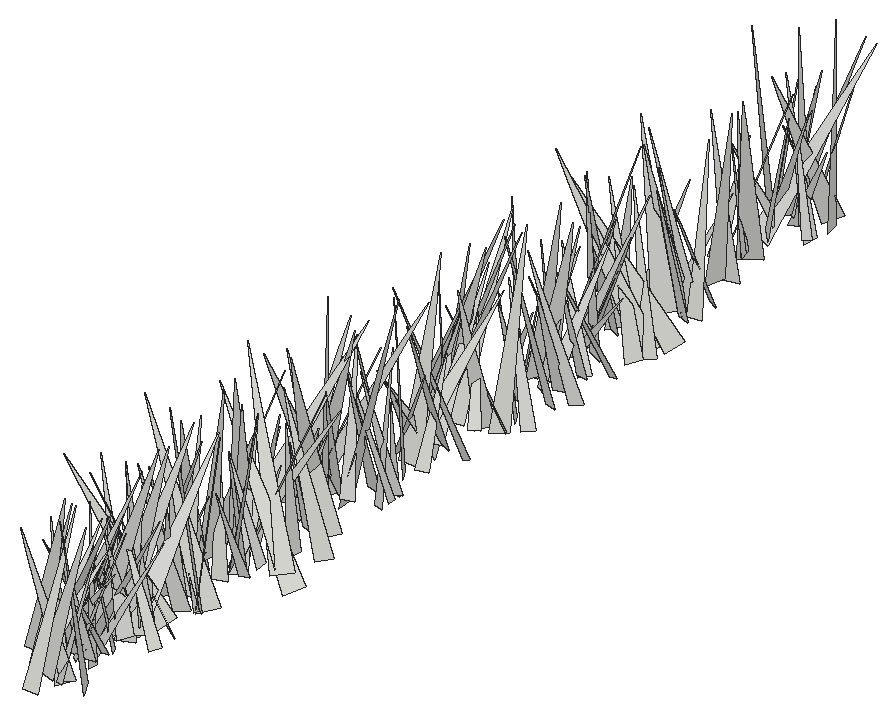
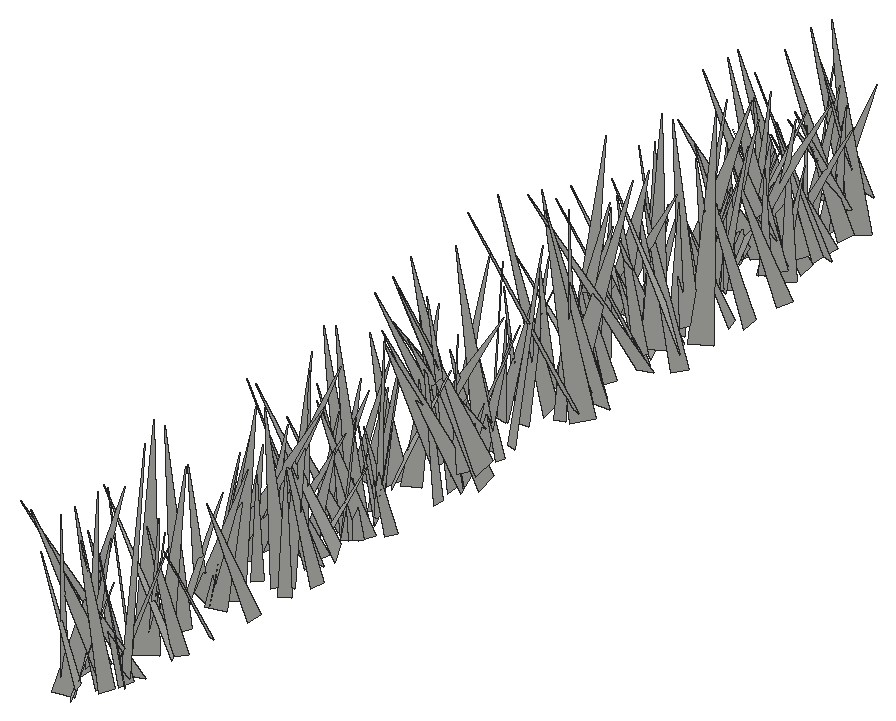
# SketchUp Ruby script. Lengths in inches.
U = 1.inch
M = Sketchup.active_model
def pt(a) = Geom::Point3d.new(a.map { |v| v * U })
def face(e, loops, mat)
  f = e.add_face(loops[0].map { |a| pt(a) })
  loops[1..].each { |l| e.add_face(l.map { |a| pt(a) }).erase! }
  f.material = f.back_material = mat if mat
  f
end
# faces: each face lists its corners as indices into pts; further lists are holes
def faces(e, pts, list, mat = nil) = list.each { |f| face(e, (f[0].is_a?(Array) ? f : [f]).map { |l| l.map { |i| pts[i] } }, mat) }
# xy, xz, yz: faces in a plane at the given z, y or x. An outline is a flat list of corners, or four numbers for a rectangle; further outlines are holes
def ring(l) = l.size == 4 ? [[l[0], l[1]], [l[2], l[1]], [l[2], l[3]], [l[0], l[3]]] : l.each_slice(2).to_a
def flat(e, list, mat, &to3) = list.each { |f| face(e, (f[0].is_a?(Array) ? f : [f]).map { |l| ring(l).map { |u, v| to3.(u, v) } }, mat) }
def xy(e, z, list, mat = nil) = flat(e, list, mat) { |x, y| [x, y, z] }
def xz(e, y, list, mat = nil) = flat(e, list, mat) { |x, z| [x, y, z] }
def yz(e, x, list, mat = nil) = flat(e, list, mat) { |y, z| [x, y, z] }
def lines(e, pts, list) = list.each { |a, b| e.add_line(pt(pts[a]), pt(pts[b])) }
# prism: a flat outline (further loops are holes) pulled along v
def prism(e, loops, v, mat = nil)
  f = face(e, loops, mat); d = Geom::Vector3d.new(v.map { |x| x * U })
  f.pushpull(f.normal.samedirection?(d) ? d.length : -d.length)
end
def box(e, o, s, mat = nil) = prism(e, [[o, [o[0] + s[0], o[1], o[2]], [o[0] + s[0], o[1] + s[1], o[2]], [o[0], o[1] + s[1], o[2]]]], [0, 0, s[2]], mat)
def at(x, y, z, deg = 0) = Geom::Transformation.translation(pt([x, y, z])) * Geom::Transformation.rotation(ORIGIN, Z_AXIS, deg.degrees)
def axes(o, x, y, z) = Geom::Transformation.new([*x, 0, *y, 0, *z, 0, *pt(o).to_a, 1])
def part(name) = M.definitions.add(name)
# library, detail: a bought-in or finely detailed component or shape, given as its bounding box
def library(name, o, s) = part(name).tap { |d| box(d.entities, o, s) }
def detail(e, o, s) = box(e.add_group.entities, o, s)
def put(e, d, t, mat = nil) = e.add_instance(d, t).tap { |i| i.material = mat if mat }
def group(e, t, mat = nil) = e.add_group.tap { |g| g.transformation = t; g.material = mat if mat }.entities
root = M.entities
c1 = part("fur_instance\#9")
p = [[0.8125,0,1.79],[0.67,-0.02,1.48],[0,-0.11,0],[0,0.11,0]]
faces(c1.entities,p,[[0,1,2,3]])
put(root,c1,axes([155.28,108.74,-27.1],[0.56131,-6.10589,2.64479],[-6.41112,0.21442,1.85565],[1.78167,2.69518,5.8441]))
put(root,c1,axes([156,106.33,-27.1],[0.77683,6.56918,0.32302],[6.56801,-0.79193,0.30978],[-0.34589,-0.28401,6.60769]))
put(root,c1,axes([157.04,109.05,-27.1],[-1.11932,5.12608,2.18052],[5.30702,0.30525,2.00664],[-1.6932,-2.43194,4.84799]))
put(root,c1,axes([157.4,110.48,-28.22],[-5.52938,-3.456,2.07939],[-3.45701,5.87854,0.57763],[2.07771,0.58365,6.49494]))
put(root,c1,axes([152.8,110.96,-27.1],[2.44609,-6.94499,1.47158],[-6.99231,-2.08787,1.76924],[1.22722,1.94671,7.14745]))
put(root,c1,axes([154.06,109.06,-27.1],[2.83544,5.2975,1.05869],[5.3487,-2.92083,0.29014],[-0.75876,-0.79328,6.00159]))
put(root,c1,axes([156.75,108.45,-27.1],[2.63197,4.07891,0.20518],[3.86496,-2.5665,1.44292],[-1.31973,0.61842,4.63495]))
put(root,c1,axes([155.76,110.05,-28.22],[-5.59826,1.4556,0.99849],[1.35798,5.67289,-0.65612],[1.12768,0.39476,5.74707]))
put(root,c1,axes([155.02,112.17,-27.1],[-0.84306,-4.44176,0.86686],[-4.52258,0.85891,0.00263],[0.16427,0.85115,4.52106]))
put(root,c1,axes([154.27,109.05,-27.1],[-0.54715,4.89077,0.10405],[4.53126,0.54616,-1.84371],[1.84341,0.10915,4.56287]))
put(root,c1,axes([156.3125,112.18,-27.1],[0.08099,-5.17118,1.20761],[-5.27072,-0.22549,-0.61212],[-0.64729,1.18913,5.13546]))
put(root,c1,axes([153.21,111.98,-27.1],[6.75875,-1.16964,0.00047],[-1.16859,-6.75255,0.29358],[0.0496,0.28936,6.85293]))
put(root,c1,axes([153.85,110.38,-27.1],[-1.09311,5.26549,0.63584],[5.05113,1.23151,-1.51458],[1.61731,-0.28736,5.16007]))
put(root,c1,axes([156.67,113.47,-27.1],[-1.81586,-4.37557,0.34615],[-4.20637,1.62778,-1.48984],[-1.25376,0.87607,4.49704]))
put(root,c1,axes([155.61,111.54,-27.1],[3.29969,3.36632,0.10349],[3.25213,-3.22241,1.12716],[-0.87548,0.71745,4.57707]))
put(root,c1,axes([155.58,112.52,-27.1],[3.89268,2.82638,0.90518],[2.67493,-3.98806,0.94914],[-1.28551,0.26015,4.71599]))
put(root,c1,axes([152.82,113.93,-27.1],[2.65844,-2.5721,0.0216],[-2.2994,-2.3625,1.67773],[1.15278,1.21916,3.2967]))
put(root,c1,axes([155.84,113.16,-28.22],[-5.50715,-0.70612,1.61288],[-1.08889,5.52799,-1.29784],[1.38358,1.53996,5.39842]))
put(root,c1,axes([155.6,115.7,-28.22],[-3.07283,-1.79032,0.75021],[-1.87261,3.10397,-0.26279],[0.51124,0.60869,3.54662]))
put(root,c1,axes([152.41,114.9,-27.1],[3.65176,6.04586,1.11201],[6.02251,-3.25936,-2.05677],[1.23222,-1.98709,6.75703]))
put(root,c1,axes([152.82,115.48,-27.1],[5.19271,0.37939,0.34653],[0.38191,-5.20401,-0.02543],[-0.34375,-0.05067,5.20649]))
put(root,c1,axes([154.72,114.96,-28.22],[3.55975,3.91646,0.08522],[3.79537,-3.41954,-1.38552],[0.97011,-0.99289,5.10792]))
put(root,c1,axes([155.55,117.68,-28.22],[3.33283,-3.55166,1.19436],[-3.37517,-3.53973,-1.10774],[-1.62758,0.06765,4.74288]))
put(root,c1,axes([158.9375,115.97,-27.1],[-4.27711,1.68369,0.0136],[1.68167,4.26988,0.26227],[-0.08344,-0.24902,4.58909]))
put(root,c1,axes([154.35,117.61,-28.22],[-3.58815,0.95471,1.93369],[1.59157,3.70529,1.12394],[1.45517,-1.69849,3.5388]))
put(root,c1,axes([153.92,116.01,-27.1],[6.10397,-4.61293,1.81963],[-4.95361,-5.80478,1.9013],[-0.22786,2.62185,7.41098]))
put(root,c1,axes([153.81,115.41,-28.22],[5.39304,-0.33096,0.39775],[-0.43435,-5.15892,1.59671],[-0.28121,1.6213,5.16187]))
put(root,c1,axes([153.73,117.42,-28.22],[3.93082,-2.70083,1.38603],[-2.7651,-4.12134,-0.18897],[-1.2529,0.6221,4.76552]))
put(root,c1,axes([156.42,115.96,-27.1],[-6.22467,1.67352,0.58559],[1.62437,6.23957,-0.56507],[0.71064,0.39649,6.42089]))
put(root,c1,axes([155.38,117.21,-28.22],[3.4619,-5.09824,2.22403],[-5.52391,-3.4582,0.67108],[-0.65172,2.22978,6.12588]))
put(root,c1,axes([157.35,119.18,-27.1],[-6.27712,3.42033,1.55819],[3.73626,5.34865,3.31076],[-0.40863,-3.63622,6.33559]))
put(root,c1,axes([156.74,117.86,-27.1],[5.59524,-0.57904,3.08549],[-0.36766,-6.38318,-0.53118],[-3.11775,-0.28642,5.59999]))
put(root,c1,axes([157.17,119.92,-28.22],[-4.1792,-5.61615,0.15739],[-5.61189,4.16336,-0.45249],[-0.26934,0.3962,6.98585]))
put(root,c1,axes([156.85,119.97,-27.1],[-4.22388,-0.55824,1.0602],[-0.01996,3.91714,1.98304],[1.19803,-1.90295,3.77099]))
put(root,c1,axes([154,118.47,-27.1],[4.37755,-6.1842,1.75356],[-6.40379,-4.01166,1.83857],[0.55746,2.47882,7.3503]))
put(root,c1,axes([156.9,116.99,-27.1],[-0.83276,5.81039,0.96307],[5.68734,0.54058,1.65638],[-1.53047,-1.15272,5.63121]))
put(root,c1,axes([154.28,119.24,-27.1],[-2.72992,2.63061,1.69887],[2.87463,2.99911,-0.02472],[1.24209,-1.1593,3.79104]))
put(root,c1,axes([154.4,117.78,-27.1],[-0.17327,7.80384,1.95788],[7.72096,0.71202,-2.15474],[2.26272,-1.83203,7.50246]))
put(root,c1,axes([152,120.01,-28.22],[4.26333,-3.02404,0.31767],[-2.97687,-4.03955,1.49732],[0.61963,1.39963,5.00788]))
put(root,c1,axes([156.96,121.24,-27.1],[0.96308,-5.75121,1.64983],[-5.7805,-1.32563,-1.24675],[-1.54408,1.37555,5.69645]))
put(root,c1,axes([155.87,117.6,-27.1],[-2.00066,7.03095,0.19663],[6.73059,1.97306,-2.06922],[2.04255,0.38513,7.01108]))
put(root,c1,axes([154.93,122.35,-27.1],[3.91329,-2.80057,0.16354],[-2.76188,-3.89534,-0.61821],[-0.49189,-0.40864,4.7723]))
put(root,c1,axes([155.8,122.39,-27.1],[1.04102,-4.92803,1.21287],[-5.07408,-1.03535,0.14838],[-0.10125,1.21771,5.0346]))
put(root,c1,axes([155.33,122.57,-27.1],[-1.95958,-4.83915,1.26512],[-4.97855,2.01787,0.00704],[0.48156,1.1699,5.22085]))
put(root,c1,axes([157.79,122.03,-27.1],[-4.59653,-5.39297,2.39685],[-5.86856,4.49796,-1.13384],[0.62378,2.57709,6.99476]))
put(root,c1,axes([158.34,122.38,-27.1],[-5.06971,5.94983,1.91077],[6.22333,4.58369,2.23904],[-0.56711,-2.88838,7.48926]))
put(root,c1,axes([157.86,121.75,-27.1],[-3.7674,-0.4134,0.34529],[-0.49063,3.64055,-0.99453],[0.22227,1.02903,3.6572]))
put(root,c1,axes([156.02,125.67,-28.22],[-5.03232,-2.4099,0.87584],[-1.92345,4.82363,2.22078],[1.6956,-1.68045,5.11859]))
put(root,c1,axes([152.14,123.56,-28.22],[6.68807,0.43229,0.66728],[0.41432,-6.71942,0.20043],[-0.67859,0.15798,6.69903]))
put(root,c1,axes([155.62,125.4,-27.1],[-2.21382,-3.77344,0.32599],[-3.76288,2.23425,0.30817],[0.43109,0.1241,4.36404]))
put(root,c1,axes([155.875,123.06,-27.1],[0.35449,6.1752,1.09899],[6.2119,-0.49795,0.79425],[-0.86782,-1.04187,6.13416]))
put(root,c1,axes([154.59,125.72,-28.22],[3.69815,0.46024,1.83595],[1.02421,-3.87534,-1.09159],[-1.5917,-1.42435,3.56322]))
put(root,c1,axes([153.07,124.3,-28.22],[3.9948,0.59542,0.26899],[0.55235,-3.96784,0.58004],[-0.34899,0.53573,3.99706]))
put(root,c1,axes([156.08,123.89,-28.22],[4.62309,3.63215,1.82021],[3.50208,-4.96051,1.00367],[-2.05939,-0.28182,5.79293]))
put(root,c1,axes([153.02,127.67,-28.22],[4.3126,-6.65441,0.44802],[-6.65528,-4.32849,-0.22777],[-0.435,0.25174,7.9264]))
put(root,c1,axes([157.32,127.48,-27.1],[0.58704,-3.79537,0.45103],[-3.78334,-0.64184,-0.47675],[-0.5428,0.36891,3.81079]))
put(root,c1,axes([153.91,127.75,-27.1],[6.97924,-1.80721,1.76653],[-1.77915,-7.19853,-0.33521],[-1.79479,0.10824,7.20163]))
put(root,c1,axes([155.84,128.07,-27.1],[5.68987,2.39384,1.65752],[2.61602,-5.80047,-0.60296],[-1.2784,-1.21517,6.14342]))
put(root,c1,axes([155.09,127.64,-28.22],[-1.15441,5.11883,1.74969],[5.40957,1.09949,0.35248],[0.0216,-1.78472,5.23554]))
put(root,c1,axes([156.03,128.94,-27.1],[-1.67476,-3.89018,1.26522],[-4.03938,1.78862,0.15259],[0.64624,1.09838,4.23261]))
put(root,c1,axes([157.33,129.25,-27.1],[-4.29082,0.07848,0.62907],[0.12494,4.3243,0.31276],[0.62151,-0.32753,4.28013]))
put(root,c1,axes([153.75,131.74,-27.1],[4.25947,-6.86655,0.67935],[-6.89421,-4.26807,0.08653],[-0.2843,0.62304,8.07992]))
put(root,c1,axes([154.02,131.65,-27.1],[3.44417,-6.15496,0.43731],[-6.17002,-3.42915,0.33004],[0.07525,0.54268,7.04535]))
put(root,c1,axes([159.93,129.55,-28.22],[-5.28258,5.45364,0.12335],[5.18528,4.96674,2.47132],[-1.69419,-1.80343,7.17917]))
put(root,c1,axes([155.55,129.04,-28.22],[3.74309,-3.05687,3.19875],[-4.02453,-4.09315,0.7978],[-1.83838,2.73658,4.76642]))
put(root,c1,axes([151.78,131.4375,-28.22],[2.36521,-5.47601,0.71506],[-5.30162,-2.03369,1.96193],[1.54624,1.40343,5.6331]))
put(root,c1,axes([159.06,129.3125,-27.1],[-3.56857,7.17935,0.49748],[7.02506,3.35468,1.97986],[-1.56176,-1.31463,7.76903]))
put(root,c1,axes([155.07,129.56,-28.22],[-2.46279,4.53865,0.90199],[4.34757,2.61941,-1.3098],[1.58479,-0.13272,4.99491]))
put(root,c1,axes([152.375,130.54,-27.1],[6.025,3.41302,0.55167],[3.40656,-6.04972,0.22351],[-0.59027,-0.07668,6.92094]))
put(root,c1,axes([154.72,130.52,-28.22],[6.48449,2.8801,0.19854],[2.8437,-6.45643,0.78158],[-0.49773,0.63448,7.05214]))
put(root,c1,axes([153.87,133,-27.1],[5.53978,-0.90724,0.62547],[-0.85463,-5.56113,-0.49688],[-0.69563,-0.39269,5.59154]))
put(root,c1,axes([156.8125,133.34,-28.22],[-4.81176,0.83188,2.6308],[1.27412,5.3609,0.63523],[2.44739,-1.15538,4.84165]))
put(root,c1,axes([154.01,132.54,-28.22],[2.6099,-2.39325,0.8726],[-2.54736,-2.4537,0.88934],[-0.00348,1.24593,3.42758]))
put(root,c1,axes([153.79,133.01,-27.1],[3.84668,4.92623,0.09388],[4.62666,-3.57049,-2.21792],[1.69428,-1.43435,5.84342]))
put(root,c1,axes([158.85,134.08,-28.22],[-2.40654,5.51072,1.54274],[5.60544,1.9331,1.83892],[-1.15197,-2.10585,5.72519]))
put(root,c1,axes([155.44,137.81,-27.1],[6.81384,-4.6319,0.82302],[-4.34734,-6.75311,-2.01405],[-1.7979,-1.22528,7.98915]))
put(root,c1,axes([155.24,136.69,-28.22],[-0.97443,-3.66118,0.75209],[-3.71136,1.03977,0.25308],[0.44234,0.6588,3.78017]))
put(root,c1,axes([157.17,136.85,-28.22],[3.76435,-5.16952,3.38659],[-5.24976,-4.76711,-1.44149],[-3.26082,1.70703,6.23028]))
put(root,c1,axes([154.72,139.375,-27.1],[4.80853,-5.64104,1.01196],[-5.19564,-4.8483,-2.3381],[-2.41883,-0.80002,7.03396]))
put(root,c1,axes([153.22,137.09,-27.1],[3.00481,-2.76961,0.12717],[-2.71494,-2.90128,0.96303],[0.56213,0.79222,3.97142]))
put(root,c1,axes([153.6,137.51,-28.22],[0.78956,-4.05986,1.16414],[-3.93825,-0.27989,1.69498],[1.52574,1.37851,3.77266]))
put(root,c1,axes([152.41,134.41,-27.1],[1.49345,8.09623,0.02611],[7.76227,-1.42429,-2.34489],[2.30146,-0.44999,7.89182]))
put(root,c1,axes([154.35,138.95,-28.22],[1.6475,-3.20979,0.84583],[-3.31321,-1.64761,0.20101],[-0.20196,0.8456,3.6023]))
put(root,c1,axes([155.5,138.28,-27.1],[-6.71268,-1.89599,2.76742],[-2.51748,6.93875,-1.3526],[2.21714,2.13833,6.8429]))
put(root,c1,axes([152.88,138.43,-28.22],[1.96643,7.28816,1.86053],[7.47956,-1.69089,-1.28167],[0.79683,-2.11408,7.43918]))
put(root,c1,axes([153.86,141.6875,-28.22],[-0.85203,-5.57664,0.61964],[-5.3803,0.98986,1.51043],[1.59225,0.36067,5.43539]))
put(root,c1,axes([152.62,140.74,-28.22],[6.79044,-4.4332,0.71146],[-4.48312,-6.76549,0.63187],[-0.24718,0.91888,8.0848]))
put(root,c1,axes([153.88,137.39,-28.22],[5.76242,3.50846,0.12226],[3.39302,-5.62636,1.53663],[-0.90093,1.2508,6.56914]))
put(root,c1,axes([156.21,139.82,-27.1],[-0.40963,5.6712,0.85204],[5.69515,0.30195,0.72827],[-0.67361,-0.89587,5.63914]))
put(root,c1,axes([155.49,143.62,-28.22],[-0.77388,-5.77446,0.46112],[-5.72229,0.83441,0.84559],[0.90132,0.33953,5.76439]))
put(root,c1,axes([155.2,140.97,-28.22],[8.05424,1.38868,1.7961],[1.29513,-8.24767,0.56905],[-1.86468,0.26973,8.15325]))
put(root,c1,axes([158.61,141.58,-27.1],[-4.94313,-1.68267,0.02369],[-1.64372,4.81198,-1.18726],[-0.36076,1.13137,5.08492]))
put(root,c1,axes([152.75,141.45,-27.1],[4.68977,6.59581,0.10077],[6.41242,-4.52929,-1.96857],[1.54784,-1.22048,7.85006]))
put(root,c1,axes([157.07,143.95,-28.22],[0.47741,-4.86513,1.33169],[-4.92648,-0.73691,-0.92606],[-1.08291,1.20759,4.79999]))
put(root,c1,axes([157.14,141.98,-28.22],[2.35955,4.93164,1.36493],[4.86886,-2.62618,1.07189],[-1.57426,-0.73054,5.36093]))
put(root,c1,axes([156.96,144.05,-28.22],[-0.48209,-3.49328,1.24378],[-3.69826,0.54426,0.09516],[0.26993,1.21786,3.5251]))
put(root,c1,axes([154.15,146.48,-28.22],[-3.66849,-5.82093,1.22872],[-5.44278,3.86666,2.06783],[2.40191,-0.1285,6.56241]))
put(root,c1,axes([157.07,144.8125,-27.1],[-5.34444,-2.84039,2.21318],[-3.30562,5.4408,-0.99979],[1.42788,1.96442,5.96919]))
put(root,c1,axes([156.45,149.73,-27.1],[-1.98153,-6.18192,0.39554],[-6.00617,2.01899,1.46585],[1.5161,-0.08133,6.32408]))
put(root,c1,axes([154.42,149.6,-28.22],[3.43107,-2.8474,0.0502],[-2.64084,-3.2106,-1.6126],[-1.06592,-1.21113,4.15686]))
put(root,c1,axes([155.6,150.16,-28.22],[-4.54437,-2.07997,0.71062],[-1.49312,4.11891,2.50752],[1.61302,-2.04715,4.32318]))
put(root,c1,axes([153.6,148.31,-28.22],[4.55769,0.07164,0.01251],[0.0727,-4.46545,-0.91231],[0.00209,-0.91239,4.46602]))
put(root,c1,axes([155.19,147.89,-28.22],[-0.77106,7.66776,2.67234],[8.04873,1.0768,-0.76736],[1.07416,-2.56446,7.66813]))
put(root,c1,axes([156.35,147.61,-28.22],[-1.99149,3.68652,0.84504],[3.6319,2.13053,-0.73532],[1.05538,-0.37542,4.12502]))
put(root,c1,axes([158.9375,149.14,-27.1],[-3.53185,-5.19128,1.06072],[-4.89285,2.7062,-3.04713],[-2.03336,2.50511,5.48984]))
put(root,c1,axes([155.11,148.36,-27.1],[-2.23637,5.81255,0.47787],[5.16217,2.21098,-2.73477],[2.71405,0.58421,5.59536]))
put(root,c1,axes([155.06,150.27,-27.1],[0.14678,4.73777,0.12743],[4.7339,-0.15274,0.22615],[-0.23006,-0.12022,4.73465]))
put(root,c1,axes([154.84,151.95,-27.1],[-3.59286,-3.26733,2.03566],[-3.70516,3.69058,-0.61592],[1.04455,1.85261,4.81713]))
put(root,c1,axes([153.31,152.77,-28.22],[3.4231,3.63538,1.50249],[3.93251,-3.11512,-1.42212],[0.09387,-2.06666,4.78656]))
put(root,c1,axes([153.35,153.07,-27.1],[6.11915,-4.70581,1.11272],[-4.83462,-5.98952,1.25659],[-0.09634,1.67568,7.61641]))
put(root,c1,axes([155.83,149.45,-27.1],[-4.8564,4.18897,0.42907],[3.70643,4.56321,-2.59917],[1.99849,1.71635,5.86314]))
put(root,c1,axes([156.01,154.84,-28.22],[4.71186,-4.25626,1.34995],[-4.06485,-4.9009,-1.26409],[-1.848,-0.07223,6.22249]))
put(root,c1,axes([152.31,151.41,-28.22],[8.13769,0.92636,1.08085],[0.65484,-8.00564,1.93114],[-1.26395,1.81658,7.95932]))
put(root,c1,axes([152.52,151.4375,-27.1],[8.0865,0.10169,1.15451],[-0.2162,-7.86244,2.20681],[-1.13864,2.21504,7.78021]))
put(root,c1,axes([153.6,153.15,-28.22],[7.00703,0.38351,2.14023],[0.30488,-7.32356,0.31416],[-2.15283,0.21111,7.01048]))
put(root,c1,axes([156.87,152.54,-27.1],[-2.11834,3.44874,0.2067],[3.45458,2.11778,0.0692],[0.04913,-0.21236,4.04678]))
put(root,c1,axes([154.38,151.59,-27.1],[7.47336,0.82298,1.26079],[0.38429,-7.21504,2.43175],[-1.45575,2.3203,7.11442]))
put(root,c1,axes([153.21,155.42,-28.22],[6.22131,1.299,1.34326],[1.60809,-6.10017,-1.54868],[-0.95174,-1.81575,6.1639]))
put(root,c1,axes([157.22,155.47,-28.22],[-3.79986,-3.34827,0.10157],[-3.34083,3.7767,-0.4853],[-0.24505,0.43103,5.04126]))
put(root,c1,axes([153.34,152.29,-28.22],[7.3603,1.92647,1.4977],[1.22652,-7.03518,3.02165],[-2.10951,2.63124,6.98247]))
put(root,c1,axes([155.12,152.48,-27.1],[-6.41092,4.00729,0.82453],[3.32918,6.00061,-3.27831],[2.37798,2.40258,6.81256]))
put(root,c1,axes([157.08,154.9375,-28.22],[-6.19625,3.45387,1.64148],[3.0912,6.3638,-1.72156],[2.25127,0.76815,6.88178]))
put(root,c1,axes([156.95,156.92,-28.22],[-4.18009,-2.38384,1.39005],[-2.61185,4.23208,-0.59649],[0.8906,1.22265,4.77494]))
put(root,c1,axes([155.72,159.07,-28.22],[0.47232,-5.02453,0.37853],[-5.03579,-0.45765,0.20889],[0.17316,0.39615,5.04235]))
put(root,c1,axes([158.5,156.3,-28.22],[-1.63602,4.97918,0.62205],[4.87533,1.42244,1.43652],[-1.18757,-1.0199,5.04036]))
put(root,c1,axes([157.61,159.76,-28.22],[-2.90009,-5.61636,1.60668],[-5.82709,2.65472,-1.23809],[-0.41218,1.98605,6.19848]))
put(root,c1,axes([155.03,159.6,-28.22],[-6.66859,-2.01923,2.71074],[-2.32845,7.09045,-0.44648],[2.45024,1.24248,6.95328]))
put(root,c1,axes([156.78,161.87,-28.22],[1.17594,-4.92519,0.34785],[-4.93492,-1.18388,-0.07952],[-0.1583,0.31979,5.06301]))
put(root,c1,axes([152.9,160.84,-28.22],[2.68666,-2.71893,0.01615],[-2.65256,-2.616,0.85524],[0.59729,0.61233,3.72549]))
put(root,c1,axes([154.74,160.13,-28.22],[3.30994,1.56111,0.94089],[1.62723,-3.40964,-0.0672],[-0.82125,-0.46405,3.659]))
put(root,c1,axes([158.75,161.09,-28.22],[-1.11932,5.12608,2.18052],[5.30702,0.30525,2.00664],[-1.6932,-2.43194,4.84799]))
put(root,c1,axes([154.34,162.39,-28.22],[7.05562,-2.47543,1.6862],[-2.53392,-7.23407,-0.01726],[-1.59697,0.54154,7.47725]))
put(root,c1,axes([154.51,163,-28.22],[2.44609,-6.94499,1.47158],[-6.99231,-2.08787,1.76924],[1.22722,1.94671,7.14745]))
put(root,c1,axes([155.77,161.1,-28.22],[2.83544,5.2975,1.05869],[5.3487,-2.92083,0.29014],[-0.75876,-0.79328,6.00159]))
put(root,c1,axes([153.9,162.14,-28.22],[3.72107,-3.56028,1.90501],[-4.03778,-3.30047,1.71878],[-0.03061,2.5656,4.85467]))
put(root,c1,axes([155.63,162.6,-28.22],[-4.56501,-1.69942,1.47091],[-1.97129,4.62695,-0.77219],[1.07964,1.26263,4.80947]))
put(root,c1,axes([156.73,164.22,-28.22],[-0.84306,-4.44176,0.86686],[-4.52258,0.85891,0.00263],[0.16427,0.85115,4.52106]))
put(root,c1,axes([156.21,163.65,-28.22],[-3.00148,-2.27694,0.1564],[-2.20162,2.82047,-1.1898],[-0.60148,1.03841,3.57459]))
put(root,c1,axes([155.56,162.42,-28.22],[-1.09311,5.26549,0.63584],[5.05113,1.23151,-1.51458],[1.61731,-0.28736,5.16007]))
put(root,c1,axes([158.38,165.51,-28.22],[-1.81586,-4.37557,0.34615],[-4.20637,1.62778,-1.48984],[-1.25376,0.87607,4.49704]))
put(root,c1,axes([156.85,164.42,-28.22],[-1.55107,4.41542,0.77186],[4.34501,1.28043,1.40671],[-1.10114,-1.16708,4.46351]))
put(root,c1,axes([154.53,165.97,-28.22],[2.65844,-2.5721,0.0216],[-2.2994,-2.3625,1.67773],[1.15278,1.21916,3.2967]))
put(root,c1,axes([155.64,166.9375,-28.22],[2.87262,5.81566,3.24646],[6.49078,-3.23727,0.05584],[-1.49368,-2.88298,6.48619]))
put(root,c1,axes([154.12,166.9375,-28.22],[3.65176,6.04586,1.11201],[6.02251,-3.25936,-2.05677],[1.23222,-1.98709,6.75703]))
put(root,c1,axes([154.53,167.52,-28.22],[5.19271,0.37939,0.34653],[0.38191,-5.20401,-0.02543],[-0.34375,-0.05067,5.20649]))
put(root,c1,axes([154.19,164.93,-28.22],[7.12213,3.78972,1.00867],[3.4176,-7.02352,2.25704],[-1.92338,1.55314,7.74548]))
put(root,c1,axes([158.21,169.54,-28.22],[-7.92246,2.32052,1.49756],[2.68865,7.5204,2.57051],[0.63138,-2.90715,7.84491]))
put(root,c1,axes([154.03,170.58,-28.22],[-1.3783,-7.92591,0.91068],[-7.76861,1.54372,1.6777],[1.81604,0.58822,7.86798]))
put(root,c1,axes([152.5,169.25,-28.22],[5.32067,-0.59583,0.38531],[-0.58759,-5.33383,-0.13414],[-0.39777,-0.09079,5.35224]))
put(root,c1,axes([158.14,168,-28.22],[-6.22467,1.67352,0.58559],[1.62437,6.23957,-0.56507],[0.71064,0.39649,6.42089]))
put(root,c1,axes([159.06,171.22,-28.22],[-6.27712,3.42033,1.55819],[3.73626,5.34865,3.31076],[-0.40863,-3.63622,6.33559]))
put(root,c1,axes([158.61,169.03,-28.22],[-0.83276,5.81039,0.96307],[5.68734,0.54058,1.65638],[-1.53047,-1.15272,5.63121]))
put(root,c1,axes([153.2,171.83,-28.22],[1.84889,-3.8875,0.07331],[-3.87281,-1.83403,0.41727],[0.34554,0.24513,4.2845]))
put(root,c1,axes([154.25,170.89,-28.22],[5.43979,-3.16023,1.66658],[-3.30816,-5.60189,0.17546],[-1.34931,0.9938,6.28869]))
put(root,c1,axes([155.99,171.28,-28.22],[-2.72992,2.63061,1.69887],[2.87463,2.99911,-0.02472],[1.24209,-1.1593,3.79104]))
put(root,c1,axes([157.04,174.62,-28.22],[-1.95958,-4.83915,1.26512],[-4.97855,2.01787,0.00704],[0.48156,1.1699,5.22085]))
put(root,c1,axes([155.58,174.46,-28.22],[-5.4764,4.5647,2.90915],[5.14181,5.68019,0.76664],[1.69155,-2.48788,7.08799]))
put(root,c1,axes([155.76,176.01,-28.22],[2.81422,-5.9892,1.8303],[-5.99838,-3.15452,-1.09945],[-1.79999,1.14839,6.52546]))
put(root,c1,axes([156.58,175.36,-28.22],[-4.89111,-2.11302,1.38613],[-2.21595,5.03778,-0.13961],[1.21481,0.68196,5.3262]))
put(root,c1,axes([157.33,177.44,-28.22],[-2.21382,-3.77344,0.32599],[-3.76288,2.23425,0.30817],[0.43109,0.1241,4.36404]))
put(root,c1,axes([157.26,175.6,-28.22],[-0.37721,6.24874,2.25952],[6.16262,-0.51732,2.45945],[-2.4848,-2.23161,5.75674]))
put(root,c1,axes([152.94,175.39,-28.22],[4.54007,-1.04122,1.07478],[-1.33062,-4.37982,1.37772],[-0.68465,1.60765,4.44952]))
put(root,c1,axes([157.59,175.1,-28.22],[0.35449,6.1752,1.09899],[6.2119,-0.49795,0.79425],[-0.86782,-1.04187,6.13416]))
put(root,c1,axes([155.625,179.79,-28.22],[6.97924,-1.80721,1.76653],[-1.77915,-7.19853,-0.33521],[-1.79479,0.10824,7.20163]))
put(root,c1,axes([153.52,179.23,-28.22],[1.90499,3.12749,0.05078],[3.06447,-1.8542,-0.76405],[0.62675,-0.43991,3.5814]))
put(root,c1,axes([156.38,180.62,-28.22],[-0.07394,-6.12578,2.47714],[-6.56947,-0.19789,-0.68546],[-0.70961,2.47033,6.08776]))
put(root,c1,axes([155.46,183.79,-28.22],[4.25947,-6.86655,0.67935],[-6.89421,-4.26807,0.08653],[-0.2843,0.62304,8.07992]))
put(root,c1,axes([156.08,182.3,-27.1],[-3.70453,-1.18645,1.17686],[-1.32576,3.8289,-0.31316],[1.01735,0.66938,3.87726]))
put(root,c1,axes([153.63,182.42,-28.22],[-1.54169,4.36128,2.00643],[4.43238,2.10262,-1.16464],[1.84406,-1.40768,4.47674]))
put(root,c1,axes([155.93,182.54,-27.1],[-4.75488,-0.89522,1.48594],[-1.16705,4.85843,-0.80746],[1.28353,1.10117,4.77057]))
put(root,c1,axes([154.08,182.58,-28.22],[6.025,3.41302,0.55167],[3.40656,-6.04972,0.22351],[-0.59027,-0.07668,6.92094]))
put(root,c1,axes([155.54,185.43,-27.1],[4.29125,3.34973,1.68987],[3.74545,-3.97458,-1.63261],[-0.21889,-2.33948,5.19327]))
put(root,c1,axes([154.88,187.22,-27.1],[-4.05266,-1.43323,0.72397],[-1.06557,3.87082,1.69814],[1.20119,-1.40176,3.94899]))
put(root,c1,axes([153.71,188.16,-27.1],[-3.953,-6.85404,2.35159],[-6.87911,4.39144,1.23577],[2.27722,1.36799,7.81517]))
put(root,c1,axes([157.96,186.66,-27.1],[-0.43735,3.78387,0.74816],[3.7266,0.2203,1.06426],[-0.99494,-0.83814,3.65736]))
put(root,c1,axes([154,187.77,-28.22],[5.3173,-1.56529,0.48292],[-1.59322,-5.32309,0.28875],[-0.38078,0.41424,5.53538]))
put(root,c1,axes([156.43,191.41,-28.22],[4.80853,-5.64104,1.01196],[-5.19564,-4.8483,-2.3381],[-2.41883,-0.80002,7.03396]))
put(root,c1,axes([157.04,188.19,-28.22],[-5.94659,0.26274,1.16381],[0.1992,6.05181,-0.34844],[1.17635,0.30341,5.94219]))
put(root,c1,axes([154.93,189.13,-28.22],[3.00481,-2.76961,0.12717],[-2.71494,-2.90128,0.96303],[0.56213,0.79222,3.97142]))
put(root,c1,axes([154.24,187.68,-28.22],[3.86177,3.77021,1.4507],[3.73701,-4.09632,0.69796],[-1.5342,-0.48777,5.35169]))
put(root,c1,axes([156.37,188.45,-27.1],[-6.67663,-0.80436,2.4344],[-1.05353,7.05179,-0.55944],[2.33738,0.88086,6.7016]))
put(root,c1,axes([154.84,188.74,-27.1],[2.00613,4.44684,1.43472],[4.67253,-1.91449,-0.59961],[-0.01581,-1.5549,4.84142]))
put(root,c1,axes([154.12,186.45,-28.22],[1.49345,8.09623,0.02611],[7.76227,-1.42429,-2.34489],[2.30146,-0.44999,7.89182]))
put(root,c1,axes([153.21,190.76,-27.1],[6.29896,-1.22347,0.37639],[-1.1888,-6.29213,-0.55798],[-0.47466,-0.47719,6.39237]))
put(root,c1,axes([155.63,191.6,-28.22],[-3.41692,-2.65793,0.41527],[-2.50813,3.39027,1.06197],[0.9728,-0.5949,4.19669]))
put(root,c1,axes([155.03,188.73,-27.1],[6.92746,0.46404,1.30725],[0.06508,-6.75935,2.05449],[-1.38564,2.00246,6.63205]))
put(root,c1,axes([157.21,190.32,-28.22],[-6.71268,-1.89599,2.76742],[-2.51748,6.93875,-1.3526],[2.21714,2.13833,6.8429]))
put(root,c1,axes([155.05,191.54,-27.1],[4.65489,2.00226,0.76997],[2.06003,-4.68544,-0.26978],[-0.59848,-0.55448,5.06006]))
